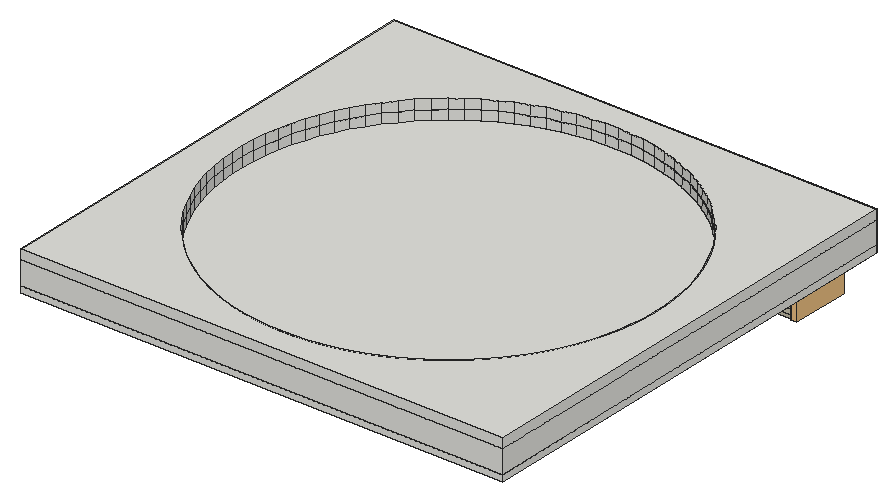
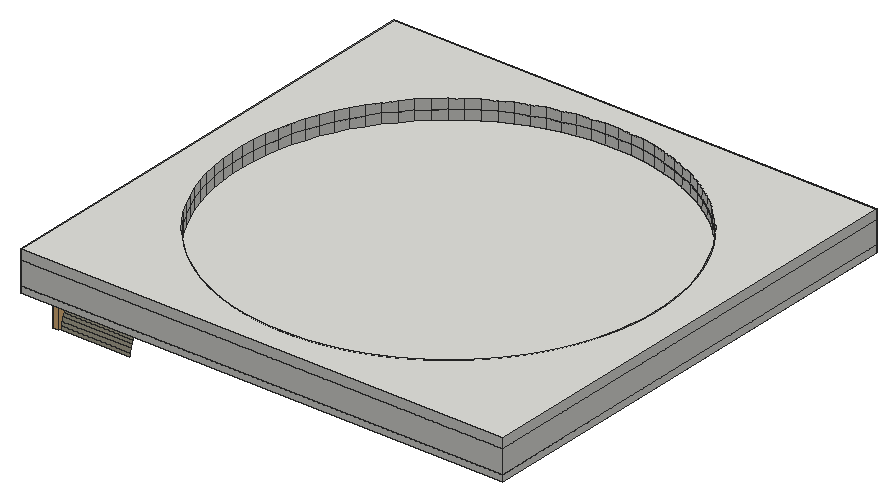
# SketchUp Ruby script. Lengths in inches.
U = 1.inch
M = Sketchup.active_model
def pt(a) = Geom::Point3d.new(a.map { |v| v * U })
def face(e, loops, mat)
  f = e.add_face(loops[0].map { |a| pt(a) })
  loops[1..].each { |l| e.add_face(l.map { |a| pt(a) }).erase! }
  f.material = f.back_material = mat if mat
  f
end
# faces: each face lists its corners as indices into pts; further lists are holes
def faces(e, pts, list, mat = nil) = list.each { |f| face(e, (f[0].is_a?(Array) ? f : [f]).map { |l| l.map { |i| pts[i] } }, mat) }
# xy, xz, yz: faces in a plane at the given z, y or x. An outline is a flat list of corners, or four numbers for a rectangle; further outlines are holes
def ring(l) = l.size == 4 ? [[l[0], l[1]], [l[2], l[1]], [l[2], l[3]], [l[0], l[3]]] : l.each_slice(2).to_a
def flat(e, list, mat, &to3) = list.each { |f| face(e, (f[0].is_a?(Array) ? f : [f]).map { |l| ring(l).map { |u, v| to3.(u, v) } }, mat) }
def xy(e, z, list, mat = nil) = flat(e, list, mat) { |x, y| [x, y, z] }
def xz(e, y, list, mat = nil) = flat(e, list, mat) { |x, z| [x, y, z] }
def yz(e, x, list, mat = nil) = flat(e, list, mat) { |y, z| [x, y, z] }
def lines(e, pts, list) = list.each { |a, b| e.add_line(pt(pts[a]), pt(pts[b])) }
# prism: a flat outline (further loops are holes) pulled along v
def prism(e, loops, v, mat = nil)
  f = face(e, loops, mat); d = Geom::Vector3d.new(v.map { |x| x * U })
  f.pushpull(f.normal.samedirection?(d) ? d.length : -d.length)
end
def box(e, o, s, mat = nil) = prism(e, [[o, [o[0] + s[0], o[1], o[2]], [o[0] + s[0], o[1] + s[1], o[2]], [o[0], o[1] + s[1], o[2]]]], [0, 0, s[2]], mat)
def at(x, y, z, deg = 0) = Geom::Transformation.translation(pt([x, y, z])) * Geom::Transformation.rotation(ORIGIN, Z_AXIS, deg.degrees)
def axes(o, x, y, z) = Geom::Transformation.new([*x, 0, *y, 0, *z, 0, *pt(o).to_a, 1])
def part(name) = M.definitions.add(name)
# library, detail: a bought-in or finely detailed component or shape, given as its bounding box
def library(name, o, s) = part(name).tap { |d| box(d.entities, o, s) }
def detail(e, o, s) = box(e.add_group.entities, o, s)
def put(e, d, t, mat = nil) = e.add_instance(d, t).tap { |i| i.material = mat if mat }
def group(e, t, mat = nil) = e.add_group.tap { |g| g.transformation = t; g.material = mat if mat }.entities
root = M.entities
M.materials.add("Tafisa-Terrarossa-PM780-4K").color = [148, 117, 107]
M.materials.add("Uniboard-L19-Putty-4K").color = [187, 181, 160]
c1 = library("Group\#28",[-0.5,-0.5,0],[2,18,8.5])
c2 = library("Group\#13",[-0.5,-0.5,0],[87.5,1,2])
c3 = library("Group\#14",[-0.5,-0.5,0],[1,108.03,2])
c4 = library("Group\#15",[-0.5,-0.5,0],[1,108.03,2])
c5 = library("Group\#16",[-0.5,-0.5,0],[87.5,1,2])
xy(root,117.88,[[119.53,40.36,120,54.5]],"Tafisa-Terrarossa-PM780-4K")
xy(root,117.88,[[119.29,20.22,120,38.24],[119.29,38.36,120,40.36],[119.29,54.5,119.53,56.5],[119.29,56.62,120,74.5],[119.29,74.62,120,92.5],
  [120,118.5,120.71,139.38]],"Uniboard-L19-Putty-4K")
xy(root,118,[[[0,0,148.5,144],[24.99,20.22,98.51,20.22,100.1875,20.375,101.56,20.83,102.625,21.6,103.39,22.66,103.85,24.04,104,25.72,104,119.76,103.85,121.4375,103.39,122.81,102.625,123.875,101.56,124.64,100.1875,125.1,98.51,125.25,24.99,125.25,23.3125,125.1,21.94,124.64,20.875,123.875,20.11,122.81,19.65,121.4375,19.5,119.76,19.5,25.72,19.65,24.04,20.11,22.66,20.875,21.6,21.94,20.83,23.3125,20.375]]])
xy(root,118,[[120,20.22,144,20.22,144,139.5,120.71,139.5,120.71,118.5,120,118.5,120,118.38,119.96,118.38,119.96,92.62,120,92.62],[119.53,54.5,120,56.5]],"Uniboard-L19-Putty-4K")
xy(root,120,[[[0,0,148.5,144],[18.5,19.22,105,126.25]],[18.5,19.22,19.5,126.25],[19.5,19.22,104,20.22],[104,19.22,105,125.25],[19.5,20.22,24.99,20.22,23.3125,20.375,21.94,20.83,20.875,21.6,20.11,22.66,19.65,24.04,19.5,25.72],
  [98.51,20.22,104,20.22,104,25.72,103.85,24.04,103.39,22.66,102.625,21.6,101.56,20.83,100.1875,20.375],[19.5,119.76,19.65,121.4375,20.11,122.81,20.875,123.875,21.94,124.64,23.3125,125.1,24.99,125.25,19.5,125.25],[104,119.76,104,125.25,98.51,125.25,100.1875,125.1,101.56,124.64,102.625,123.875,103.39,122.81,103.85,121.4375],[19.5,125.25,105,126.25]])
xy(root,122,[[18.5,19.22,105,126.25]])
xy(root,124,[[73.42,7.76,77.45,7.83,81.47,8.16,85.47,8.74,89.42,9.57,93.31,10.64,97.125,11.96,100.85,13.51,104.47,15.3,107.97,17.31,111.34,19.53,114.56,21.97,117.62,24.6,120.51,27.41,123.22,30.41,125.73,33.5625,128.05,36.87,130.15,40.32,132.02,43.89,133.68,47.57,135.09,51.35,136.27,55.21,137.2,59.14,137.88,63.12,138.32,67.13,138.49,71.17,138.42,75.2,138.09,79.22,137.51,83.22,136.68,87.17,135.61,91.06,134.29,94.875,132.74,98.6,130.95,102.22,128.94,105.72,126.72,109.09,124.28,112.31,121.65,115.37,118.84,118.26,115.84,120.97,112.6875,123.48,109.38,125.8,105.93,127.9,102.36,129.77,98.68,131.43,94.9,132.84,91.04,134.02,87.11,134.95,83.13,135.63,79.12,136.07,75.08,136.24,71.05,136.17,67.03,135.84,63.03,135.26,59.08,134.43,55.19,133.36,51.375,132.04,47.65,130.49,44.03,128.7,40.53,126.69,37.16,124.47,33.94,122.03,30.88,119.4,27.99,116.59,25.28,113.59,22.77,110.4375,20.45,107.13,18.35,103.68,16.48,100.11,14.82,96.43,13.41,92.65,12.23,88.79,11.3,84.86,10.62,80.88,10.18,76.87,10.01,72.83,10.08,68.8,10.41,64.78,10.99,60.78,11.82,56.83,12.89,52.94,14.21,49.125,15.76,45.4,17.55,41.78,19.56,38.28,21.78,34.91,24.22,31.69,26.85,28.63,29.66,25.74,32.66,23.03,35.8125,20.52,39.12,18.2,42.57,16.1,46.14,14.23,49.82,12.57,53.6,11.16,57.46,9.98,61.39,9.05,65.37,8.37,69.38,7.93]])
xy(root,127,[[[0,0,148.5,144],[73.42,7.76,77.45,7.83,81.47,8.16,85.47,8.74,89.42,9.57,93.31,10.64,97.125,11.96,100.85,13.51,104.47,15.3,107.97,17.31,111.34,19.53,114.56,21.97,117.62,24.6,120.51,27.41,123.22,30.41,125.73,33.5625,128.05,36.87,130.15,40.32,132.02,43.89,133.68,47.57,135.09,51.35,136.27,55.21,137.2,59.14,137.88,63.12,138.32,67.13,138.49,71.17,138.42,75.2,138.09,79.22,137.51,83.22,136.68,87.17,135.61,91.06,134.29,94.875,132.74,98.6,130.95,102.22,128.94,105.72,126.72,109.09,124.28,112.31,121.65,115.37,118.84,118.26,115.84,120.97,112.6875,123.48,109.38,125.8,105.93,127.9,102.36,129.77,98.68,131.43,94.9,132.84,91.04,134.02,87.11,134.95,83.13,135.63,79.12,136.07,75.08,136.24,71.05,136.17,67.03,135.84,63.03,135.26,59.08,134.43,55.19,133.36,51.375,132.04,47.65,130.49,44.03,128.7,40.53,126.69,37.16,124.47,33.94,122.03,30.88,119.4,27.99,116.59,25.28,113.59,22.77,110.4375,20.45,107.13,18.35,103.68,16.48,100.11,14.82,96.43,13.41,92.65,12.23,88.79,11.3,84.86,10.62,80.88,10.18,76.87,10.01,72.83,10.08,68.8,10.41,64.78,10.99,60.78,11.82,56.83,12.89,52.94,14.21,49.125,15.76,45.4,17.55,41.78,19.56,38.28,21.78,34.91,24.22,31.69,26.85,28.63,29.66,25.74,32.66,23.03,35.8125,20.52,39.12,18.2,42.57,16.1,46.14,14.23,49.82,12.57,53.6,11.16,57.46,9.98,61.39,9.05,65.37,8.37,69.38,7.93]]])
xy(root,130,[[[0,0,148.5,144],[73.42,7.76,69.38,7.93,65.37,8.37,61.39,9.05,57.46,9.98,53.6,11.16,49.82,12.57,46.14,14.23,42.57,16.1,39.12,18.2,35.8125,20.52,32.66,23.03,29.66,25.74,26.85,28.63,24.22,31.69,21.78,34.91,19.56,38.28,17.55,41.78,15.76,45.4,14.21,49.125,12.89,52.94,11.82,56.83,10.99,60.78,10.41,64.78,10.08,68.8,10.01,72.83,10.18,76.87,10.62,80.88,11.3,84.86,12.23,88.79,13.41,92.65,14.82,96.43,16.48,100.11,18.35,103.68,20.45,107.13,22.77,110.4375,25.28,113.59,27.99,116.59,30.88,119.4,33.94,122.03,37.16,124.47,40.53,126.69,44.03,128.7,47.65,130.49,51.375,132.04,55.19,133.36,59.08,134.43,63.03,135.26,67.03,135.84,71.05,136.17,75.08,136.24,79.12,136.07,83.13,135.63,87.11,134.95,91.04,134.02,94.9,132.84,98.68,131.43,102.36,129.77,105.93,127.9,109.38,125.8,112.6875,123.48,115.84,120.97,118.84,118.26,121.65,115.37,124.28,112.31,126.72,109.09,128.94,105.72,130.95,102.22,132.74,98.6,134.29,94.875,135.61,91.06,136.68,87.17,137.51,83.22,138.09,79.22,138.42,75.2,138.49,71.17,138.32,67.13,137.88,63.12,137.2,59.14,136.27,55.21,135.09,51.35,133.68,47.57,132.02,43.89,130.15,40.32,128.05,36.87,125.73,33.5625,123.22,30.41,120.51,27.41,117.62,24.6,114.56,21.97,111.34,19.53,107.97,17.31,104.47,15.3,100.85,13.51,97.125,11.96,93.31,10.64,89.42,9.57,85.47,8.74,81.47,8.16,77.45,7.83]]])
xz(root,0,[[0,118,148.5,120],[0,120,148.5,127],[0,127,148.5,130]])
xz(root,20.22,[[24.99,118,98.51,120]])
xz(root,54.5,[[119.53,117.88,120,118]],"Tafisa-Terrarossa-PM780-4K")
xz(root,118.5,[[120,117.88,120.71,118]],"Uniboard-L19-Putty-4K")
xz(root,125.25,[[24.99,118,98.51,120]])
xz(root,144,[[0,118,148.5,120],[0,120,148.5,127],[0,127,148.5,130]])
yz(root,0,[[0,118,144,120],[0,120,144,127],[0,127,144,130]])
yz(root,19.5,[[25.72,118,119.76,120]])
yz(root,104,[[25.72,118,119.76,120]])
yz(root,119.53,[[54.5,117.88,56.5,118]],"Uniboard-L19-Putty-4K")
yz(root,120.71,[[118.5,117.88,139.38,118]],"Uniboard-L19-Putty-4K")
yz(root,148.5,[[0,118,144,120],[0,120,144,127],[0,127,144,130]])
p = [[120,120.57,108.61],[141.83,120.57,108.61],[141.83,120.5,107.5],[120,120.5,107.5],[120,137.5,107.5],[141.83,137.5,107.5],
  [141.83,137.43,108.61],[120,137.43,108.61],[120,120.79,109.7],[141.83,120.79,109.7],[141.83,137.21,109.7],[120,137.21,109.7],
  [120,121.15,110.75],[141.83,121.15,110.75],[141.83,136.85,110.75],[120,136.85,110.75],[120,121.64,111.75],[141.83,121.64,111.75],
  [141.83,136.36,111.75],[120,136.36,111.75],[120,122.26,112.67],[141.83,122.26,112.67],[141.83,135.74,112.67],[120,135.74,112.67],
  [120,122.99,113.51],[141.83,122.99,113.51],[141.83,135.01,113.51],[120,135.01,113.51],[120,123.83,114.24],[141.83,123.83,114.24],
  [141.83,134.17,114.24],[120,134.17,114.24],[120,124.75,114.86],[141.83,124.75,114.86],[141.83,133.25,114.86],[120,133.25,114.86],
  [120,125.75,115.35],[141.83,125.75,115.35],[141.83,132.25,115.35],[120,132.25,115.35],[120,126.8,115.71],[141.83,126.8,115.71],
  [141.83,131.2,115.71],[120,131.2,115.71],[120,127.89,115.93],[141.83,127.89,115.93],[141.83,130.11,115.93],[120,130.11,115.93],
  [120,129,116],[141.83,129,116],[24.99,20.22,120],[24.99,20.22,118],[23.3125,20.375,118],[23.3125,20.375,120],
  [100.1875,20.375,120],[100.1875,20.375,118],[98.51,20.22,118],[98.51,20.22,120],[21.94,20.83,118],[21.94,20.83,120],
  [101.56,20.83,120],[101.56,20.83,118],[20.875,21.6,118],[20.875,21.6,120],[102.625,21.6,120],[102.625,21.6,118],
  [20.11,22.66,118],[20.11,22.66,120],[103.39,22.66,120],[103.39,22.66,118],[19.65,24.04,118],[19.65,24.04,120],
  [103.85,24.04,120],[103.85,24.04,118],[19.5,25.72,118],[19.5,25.72,120],[104,25.72,120],[104,25.72,118],
  [19.5,119.76,120],[19.5,119.76,118],[19.65,121.4375,118],[19.65,121.4375,120],[104,119.76,118],[104,119.76,120],
  [103.85,121.4375,120],[103.85,121.4375,118],[20.11,122.81,118],[20.11,122.81,120],[103.39,122.81,120],[103.39,122.81,118],
  [20.875,123.875,118],[20.875,123.875,120],[102.625,123.875,120],[102.625,123.875,118],[21.94,124.64,118],[21.94,124.64,120],
  [101.56,124.64,120],[101.56,124.64,118],[23.3125,125.1,118],[23.3125,125.1,120],[100.1875,125.1,120],[100.1875,125.1,118],
  [24.99,125.25,118],[24.99,125.25,120],[98.51,125.25,120],[98.51,125.25,118],[73.42,7.76,124],[69.38,7.93,124],
  [69.38,7.93,127],[73.42,7.76,127],[77.45,7.83,124],[77.45,7.83,127],[81.47,8.16,124],[81.47,8.16,127],
  [65.37,8.37,124],[65.37,8.37,127],[85.47,8.74,124],[85.47,8.74,127],[61.39,9.05,124],[61.39,9.05,127],
  [89.42,9.57,124],[89.42,9.57,127],[57.46,9.98,124],[57.46,9.98,127],[93.31,10.64,124],[93.31,10.64,127],
  [53.6,11.16,124],[53.6,11.16,127],[97.125,11.96,124],[97.125,11.96,127],[49.82,12.57,124],[49.82,12.57,127],
  [100.85,13.51,124],[100.85,13.51,127],[46.14,14.23,124],[46.14,14.23,127],[104.47,15.3,124],[104.47,15.3,127],
  [42.57,16.1,124],[42.57,16.1,127],[107.97,17.31,124],[107.97,17.31,127],[39.12,18.2,124],[39.12,18.2,127],
  [111.34,19.53,124],[111.34,19.53,127],[35.8125,20.52,124],[35.8125,20.52,127],[114.56,21.97,124],[114.56,21.97,127],
  [32.66,23.03,124],[32.66,23.03,127],[117.62,24.6,124],[117.62,24.6,127],[29.66,25.74,124],[29.66,25.74,127],
  [120.51,27.41,124],[120.51,27.41,127],[26.85,28.63,124],[26.85,28.63,127],[123.22,30.41,124],[123.22,30.41,127],
  [24.22,31.69,124],[24.22,31.69,127],[125.73,33.5625,124],[125.73,33.5625,127],[21.78,34.91,124],[21.78,34.91,127],
  [128.05,36.87,124],[128.05,36.87,127],[19.56,38.28,124],[19.56,38.28,127],[130.15,40.32,124],[130.15,40.32,127],
  [17.55,41.78,124],[17.55,41.78,127],[132.02,43.89,124],[132.02,43.89,127],[15.76,45.4,124],[15.76,45.4,127],
  [133.68,47.57,124],[133.68,47.57,127],[14.21,49.125,124],[14.21,49.125,127],[135.09,51.35,124],[135.09,51.35,127],
  [12.89,52.94,124],[12.89,52.94,127],[136.27,55.21,124],[136.27,55.21,127],[11.82,56.83,124],[11.82,56.83,127],
  [137.2,59.14,124],[137.2,59.14,127],[10.99,60.78,124],[10.99,60.78,127],[137.88,63.12,124],[137.88,63.12,127],
  [10.41,64.78,124],[10.41,64.78,127],[138.32,67.13,124],[138.32,67.13,127],[10.08,68.8,124],[10.08,68.8,127],
  [138.49,71.17,124],[138.49,71.17,127],[10.01,72.83,124],[10.01,72.83,127],[138.42,75.2,124],[138.42,75.2,127],
  [10.18,76.87,124],[10.18,76.87,127],[138.09,79.22,124],[138.09,79.22,127],[10.62,80.88,124],[10.62,80.88,127],
  [137.51,83.22,124],[137.51,83.22,127],[11.3,84.86,124],[11.3,84.86,127],[136.68,87.17,124],[136.68,87.17,127],
  [12.23,88.79,124],[12.23,88.79,127],[135.61,91.06,124],[135.61,91.06,127],[13.41,92.65,124],[13.41,92.65,127],
  [134.29,94.875,124],[134.29,94.875,127],[14.82,96.43,124],[14.82,96.43,127],[132.74,98.6,124],[132.74,98.6,127],
  [16.48,100.11,124],[16.48,100.11,127],[130.95,102.22,124],[130.95,102.22,127],[18.35,103.68,124],[18.35,103.68,127],
  [128.94,105.72,124],[128.94,105.72,127],[20.45,107.13,124],[20.45,107.13,127],[126.72,109.09,124],[126.72,109.09,127],
  [22.77,110.4375,124],[22.77,110.4375,127],[124.28,112.31,124],[124.28,112.31,127],[25.28,113.59,124],[25.28,113.59,127],
  [121.65,115.37,124],[121.65,115.37,127],[27.99,116.59,124],[27.99,116.59,127],[118.84,118.26,124],[118.84,118.26,127],
  [30.88,119.4,124],[30.88,119.4,127],[115.84,120.97,124],[115.84,120.97,127],[33.94,122.03,124],[33.94,122.03,127],
  [112.6875,123.48,124],[112.6875,123.48,127],[37.16,124.47,124],[37.16,124.47,127],[109.38,125.8,124],[109.38,125.8,127],
  [40.53,126.69,124],[40.53,126.69,127],[105.93,127.9,124],[105.93,127.9,127],[44.03,128.7,124],[44.03,128.7,127],
  [102.36,129.77,124],[102.36,129.77,127],[47.65,130.49,124],[47.65,130.49,127],[98.68,131.43,124],[98.68,131.43,127],
  [51.375,132.04,124],[51.375,132.04,127],[94.9,132.84,124],[94.9,132.84,127],[55.19,133.36,124],[55.19,133.36,127],
  [91.04,134.02,124],[91.04,134.02,127],[59.08,134.43,124],[59.08,134.43,127],[87.11,134.95,124],[87.11,134.95,127],
  [63.03,135.26,124],[63.03,135.26,127],[83.13,135.63,124],[83.13,135.63,127],[67.03,135.84,124],[67.03,135.84,127],
  [79.12,136.07,124],[79.12,136.07,127],[71.05,136.17,124],[71.05,136.17,127],[75.08,136.24,124],[75.08,136.24,127],
  [69.38,7.93,130],[73.42,7.76,130],[77.45,7.83,130],[81.47,8.16,130],[65.37,8.37,130],[85.47,8.74,130],
  [61.39,9.05,130],[89.42,9.57,130],[57.46,9.98,130],[93.31,10.64,130],[53.6,11.16,130],[97.125,11.96,130],
  [49.82,12.57,130],[100.85,13.51,130],[46.14,14.23,130],[104.47,15.3,130],[42.57,16.1,130],[107.97,17.31,130],
  [39.12,18.2,130],[111.34,19.53,130],[35.8125,20.52,130],[114.56,21.97,130],[32.66,23.03,130],[117.62,24.6,130],
  [29.66,25.74,130],[120.51,27.41,130],[26.85,28.63,130],[123.22,30.41,130],[24.22,31.69,130],[125.73,33.5625,130],
  [21.78,34.91,130],[128.05,36.87,130],[19.56,38.28,130],[130.15,40.32,130],[17.55,41.78,130],[132.02,43.89,130],
  [15.76,45.4,130],[133.68,47.57,130],[14.21,49.125,130],[135.09,51.35,130],[12.89,52.94,130],[136.27,55.21,130],
  [11.82,56.83,130],[137.2,59.14,130],[10.99,60.78,130],[137.88,63.12,130],[10.41,64.78,130],[138.32,67.13,130],
  [10.08,68.8,130],[138.49,71.17,130],[10.01,72.83,130],[138.42,75.2,130],[10.18,76.87,130],[138.09,79.22,130],
  [10.62,80.88,130],[137.51,83.22,130],[11.3,84.86,130],[136.68,87.17,130],[12.23,88.79,130],[135.61,91.06,130],
  [13.41,92.65,130],[134.29,94.875,130],[14.82,96.43,130],[132.74,98.6,130],[16.48,100.11,130],[130.95,102.22,130],
  [18.35,103.68,130],[128.94,105.72,130],[20.45,107.13,130],[126.72,109.09,130],[22.77,110.4375,130],[124.28,112.31,130],
  [25.28,113.59,130],[121.65,115.37,130],[27.99,116.59,130],[118.84,118.26,130],[30.88,119.4,130],[115.84,120.97,130],
  [33.94,122.03,130],[112.6875,123.48,130],[37.16,124.47,130],[109.38,125.8,130],[40.53,126.69,130],[105.93,127.9,130],
  [44.03,128.7,130],[102.36,129.77,130],[47.65,130.49,130],[98.68,131.43,130],[51.375,132.04,130],[94.9,132.84,130],
  [55.19,133.36,130],[91.04,134.02,130],[59.08,134.43,130],[87.11,134.95,130],[63.03,135.26,130],[83.13,135.63,130],
  [67.03,135.84,130],[79.12,136.07,130],[71.05,136.17,130],[75.08,136.24,130]]
faces(root,p,[[0,1,2,3],[4,5,6,7],[8,9,1,0],[7,6,10,11],[12,13,9,8],[11,10,14,15],[16,17,13,12],[15,14,18,19],
  [20,21,17,16],[19,18,22,23],[24,25,21,20],[23,22,26,27],[28,29,25,24],[27,26,30,31],[32,33,29,28],[31,30,34,35],
  [36,37,33,32],[35,34,38,39],[40,41,37,36],[39,38,42,43],[44,45,41,40],[43,42,46,47],[48,49,45,44],[47,46,49,48]],"Uniboard-L19-Putty-4K")
faces(root,p,[[50,51,52,53],[54,55,56,57],[53,52,58,59],[60,61,55,54],[59,58,62,63],[64,65,61,60],[63,62,66,67],[68,69,65,64],
  [67,66,70,71],[72,73,69,68],[71,70,74,75],[76,77,73,72],[78,79,80,81],[82,83,84,85],[81,80,86,87],[85,84,88,89],
  [87,86,90,91],[89,88,92,93],[91,90,94,95],[93,92,96,97],[95,94,98,99],[97,96,100,101],[99,98,102,103],[101,100,104,105],
  [106,107,108,109],[110,106,109,111],[112,110,111,113],[107,114,115,108],[116,112,113,117],[114,118,119,115],[120,116,117,121],[118,122,123,119],
  [124,120,121,125],[122,126,127,123],[128,124,125,129],[126,130,131,127],[132,128,129,133],[130,134,135,131],[136,132,133,137],[134,138,139,135],
  [140,136,137,141],[138,142,143,139],[144,140,141,145],[142,146,147,143],[148,144,145,149],[146,150,151,147],[152,148,149,153],[150,154,155,151],
  [156,152,153,157],[154,158,159,155],[160,156,157,161],[158,162,163,159],[164,160,161,165],[162,166,167,163],[168,164,165,169],[166,170,171,167],
  [172,168,169,173],[170,174,175,171],[176,172,173,177],[174,178,179,175],[180,176,177,181],[178,182,183,179],[184,180,181,185],[182,186,187,183],
  [188,184,185,189],[186,190,191,187],[192,188,189,193],[190,194,195,191],[196,192,193,197],[194,198,199,195],[200,196,197,201],[198,202,203,199],
  [204,200,201,205],[202,206,207,203],[208,204,205,209],[206,210,211,207],[212,208,209,213],[210,214,215,211],[216,212,213,217],[214,218,219,215],
  [220,216,217,221],[218,222,223,219],[224,220,221,225],[222,226,227,223],[228,224,225,229],[226,230,231,227],[232,228,229,233],[230,234,235,231],
  [236,232,233,237],[234,238,239,235],[240,236,237,241],[238,242,243,239],[244,240,241,245],[242,246,247,243],[248,244,245,249],[246,250,251,247],
  [252,248,249,253],[250,254,255,251],[256,252,253,257],[254,258,259,255],[260,256,257,261],[258,262,263,259],[264,260,261,265],[262,266,267,263],
  [268,264,265,269],[266,270,271,267],[272,268,269,273],[270,274,275,271],[276,272,273,277],[274,278,279,275],[280,276,277,281],[278,282,283,279],
  [284,280,281,285],[282,286,287,283],[288,284,285,289],[286,290,291,287],[292,288,289,293],[290,294,295,291],[296,292,293,297],[294,298,299,295],
  [300,296,297,301],[298,302,303,299],[304,300,301,305],[302,304,305,303],[306,307,109,108],[307,308,111,109],[308,309,113,111],[310,306,108,115],
  [309,311,117,113],[312,310,115,119],[311,313,121,117],[314,312,119,123],[313,315,125,121],[316,314,123,127],[315,317,129,125],[318,316,127,131],
  [317,319,133,129],[320,318,131,135],[319,321,137,133],[322,320,135,139],[321,323,141,137],[324,322,139,143],[323,325,145,141],[326,324,143,147],
  [325,327,149,145],[328,326,147,151],[327,329,153,149],[330,328,151,155],[329,331,157,153],[332,330,155,159],[331,333,161,157],[334,332,159,163],
  [333,335,165,161],[336,334,163,167],[335,337,169,165],[338,336,167,171],[337,339,173,169],[340,338,171,175],[339,341,177,173],[342,340,175,179],
  [341,343,181,177],[344,342,179,183],[343,345,185,181],[346,344,183,187],[345,347,189,185],[348,346,187,191],[347,349,193,189],[350,348,191,195],
  [349,351,197,193],[352,350,195,199],[351,353,201,197],[354,352,199,203],[353,355,205,201],[356,354,203,207],[355,357,209,205],[358,356,207,211],
  [357,359,213,209],[360,358,211,215],[359,361,217,213],[362,360,215,219],[361,363,221,217],[364,362,219,223],[363,365,225,221],[366,364,223,227],
  [365,367,229,225],[368,366,227,231],[367,369,233,229],[370,368,231,235],[369,371,237,233],[372,370,235,239],[371,373,241,237],[374,372,239,243],
  [373,375,245,241],[376,374,243,247],[375,377,249,245],[378,376,247,251],[377,379,253,249],[380,378,251,255],[379,381,257,253],[382,380,255,259],
  [381,383,261,257],[384,382,259,263],[383,385,265,261],[386,384,263,267],[385,387,269,265],[388,386,267,271],[387,389,273,269],[390,388,271,275],
  [389,391,277,273],[392,390,275,279],[391,393,281,277],[394,392,279,283],[393,395,285,281],[396,394,283,287],[395,397,289,285],[398,396,287,291],
  [397,399,293,289],[400,398,291,295],[399,401,297,293],[402,400,295,299],[401,403,301,297],[404,402,299,303],[403,405,305,301],[405,404,303,305]])
put(root,c1,at(141.83,120.5,107.5),"Uniboard-L19-Putty-4K")
put(root,c2,at(18.5,126.25,120))
put(root,c3,at(18.5,19.22,120))
put(root,c4,at(105,19.22,120))
put(root,c5,at(18.5,19.22,120))
